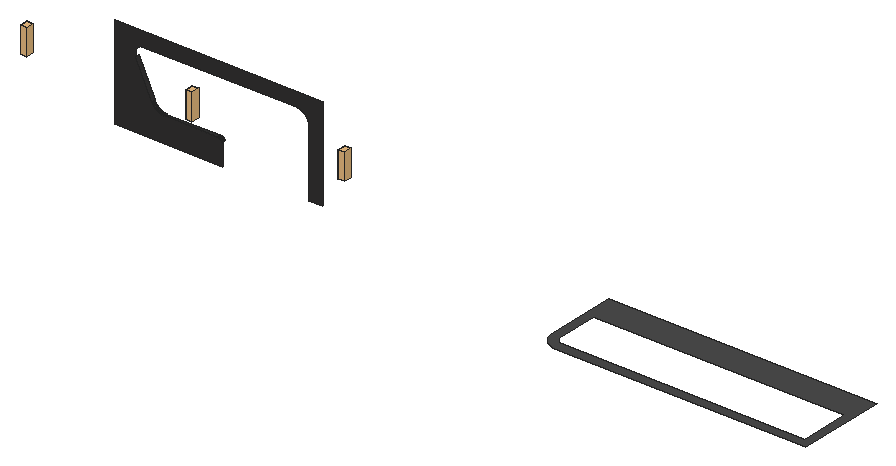
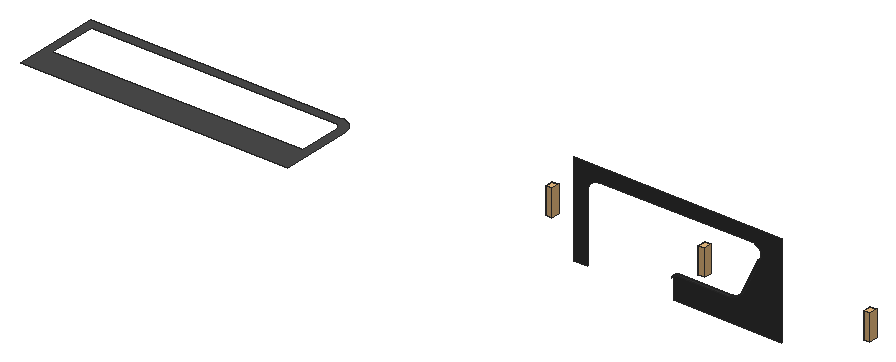
# SketchUp Ruby script. Lengths in inches.
U = 1.inch
M = Sketchup.active_model
def pt(a) = Geom::Point3d.new(a.map { |v| v * U })
def face(e, loops, mat)
  f = e.add_face(loops[0].map { |a| pt(a) })
  loops[1..].each { |l| e.add_face(l.map { |a| pt(a) }).erase! }
  f.material = f.back_material = mat if mat
  f
end
# faces: each face lists its corners as indices into pts; further lists are holes
def faces(e, pts, list, mat = nil) = list.each { |f| face(e, (f[0].is_a?(Array) ? f : [f]).map { |l| l.map { |i| pts[i] } }, mat) }
# xy, xz, yz: faces in a plane at the given z, y or x. An outline is a flat list of corners, or four numbers for a rectangle; further outlines are holes
def ring(l) = l.size == 4 ? [[l[0], l[1]], [l[2], l[1]], [l[2], l[3]], [l[0], l[3]]] : l.each_slice(2).to_a
def flat(e, list, mat, &to3) = list.each { |f| face(e, (f[0].is_a?(Array) ? f : [f]).map { |l| ring(l).map { |u, v| to3.(u, v) } }, mat) }
def xy(e, z, list, mat = nil) = flat(e, list, mat) { |x, y| [x, y, z] }
def xz(e, y, list, mat = nil) = flat(e, list, mat) { |x, z| [x, y, z] }
def yz(e, x, list, mat = nil) = flat(e, list, mat) { |y, z| [x, y, z] }
def lines(e, pts, list) = list.each { |a, b| e.add_line(pt(pts[a]), pt(pts[b])) }
# prism: a flat outline (further loops are holes) pulled along v
def prism(e, loops, v, mat = nil)
  f = face(e, loops, mat); d = Geom::Vector3d.new(v.map { |x| x * U })
  f.pushpull(f.normal.samedirection?(d) ? d.length : -d.length)
end
def box(e, o, s, mat = nil) = prism(e, [[o, [o[0] + s[0], o[1], o[2]], [o[0] + s[0], o[1] + s[1], o[2]], [o[0], o[1] + s[1], o[2]]]], [0, 0, s[2]], mat)
def at(x, y, z, deg = 0) = Geom::Transformation.translation(pt([x, y, z])) * Geom::Transformation.rotation(ORIGIN, Z_AXIS, deg.degrees)
def axes(o, x, y, z) = Geom::Transformation.new([*x, 0, *y, 0, *z, 0, *pt(o).to_a, 1])
def part(name) = M.definitions.add(name)
# library, detail: a bought-in or finely detailed component or shape, given as its bounding box
def library(name, o, s) = part(name).tap { |d| box(d.entities, o, s) }
def detail(e, o, s) = box(e.add_group.entities, o, s)
def put(e, d, t, mat = nil) = e.add_instance(d, t).tap { |i| i.material = mat if mat }
def group(e, t, mat = nil) = e.add_group.tap { |g| g.transformation = t; g.material = mat if mat }.entities
root = M.entities
M.materials.add("[Granite Dark Gray]").color = [51, 50, 50]
M.materials.add("[Stone Coursed Rough]").color = [76, 76, 76]
c1 = library("WALL LIGHT 69",[4.19,4.05,-9.63],[4.61,5.7,18.83])
xy(root,6,[[[479.6875,0,660,0,660,63,468,63,468,11.6875,468.01,11.53,468.02,11.37,468.03,11.22,468.05,10.9,468.07,10.75,468.08,10.59,468.1,10.43,468.125,10.28,468.15,10.12,468.17,9.97,468.2,9.8125,468.23,9.66,468.26,9.51,468.3,9.35,468.33,9.2,468.37,9.05,468.41,8.89,468.49,8.59,468.64,8.14,468.6875,7.99,468.74,7.85,468.8,7.7,468.85,7.55,468.91,7.41,468.97,7.26,469.04,7.12,469.1,6.98,469.17,6.83,469.45,6.27,469.53,6.14,469.61,6,469.6875,5.86,469.77,5.73,469.85,5.6,469.9375,5.46,470.02,5.33,470.2,5.07,470.29,4.95,470.38,4.82,470.48,4.69,470.58,4.57,470.67,4.45,470.77,4.33,470.98,4.09,471.08,3.97,471.1875,3.85,471.3,3.74,471.4,3.625,471.51,3.51,471.625,3.4,471.74,3.3,471.85,3.1875,471.97,3.08,472.09,2.98,472.33,2.77,472.45,2.67,472.57,2.58,472.69,2.48,472.82,2.38,472.95,2.29,473.07,2.2,473.33,2.02,473.46,1.9375,473.6,1.85,473.73,1.77,473.86,1.6875,474,1.61,474.14,1.53,474.27,1.45,474.83,1.17,474.98,1.1,475.12,1.04,475.26,0.97,475.41,0.91,475.55,0.85,475.7,0.8,475.85,0.74,475.99,0.6875,476.14,0.64,476.59,0.49,476.89,0.41,477.05,0.37,477.2,0.33,477.35,0.3,477.51,0.26,477.66,0.23,477.8125,0.2,477.97,0.17,478.12,0.15,478.28,0.125,478.43,0.1,478.59,0.08,478.75,0.07,478.9,0.05,479.22,0.03,479.37,0.02,479.53,0.01],[479.76,6,479.6875,6.01,479.61,6.01,479.45,6.03,479.37,6.03,479.29,6.04,479.22,6.05,479.14,6.0625,479.0625,6.07,478.98,6.09,478.91,6.1,478.83,6.12,478.75,6.13,478.68,6.15,478.6,6.17,478.52,6.18,478.45,6.2,478.37,6.23,478.3,6.25,478.22,6.27,478.15,6.29,478.07,6.32,478,6.34,477.92,6.37,477.78,6.43,477.7,6.46,477.42,6.58,477.35,6.62,477.28,6.65,477.07,6.77,477,6.8,476.93,6.84,476.87,6.88,476.8,6.93,476.73,6.97,476.67,7.01,476.6,7.06,476.54,7.1,476.47,7.15,476.41,7.19,476.29,7.29,476.22,7.34,476.16,7.39,476.1,7.4375,476.04,7.49,475.99,7.54,475.93,7.59,475.87,7.65,475.8125,7.7,475.76,7.76,475.7,7.8125,475.65,7.87,475.59,7.93,475.54,7.99,475.49,8.04,475.4375,8.1,475.39,8.16,475.34,8.22,475.29,8.29,475.19,8.41,475.15,8.47,475.1,8.54,475.06,8.6,475.01,8.67,474.97,8.73,474.93,8.8,474.88,8.87,474.84,8.93,474.8,9,474.77,9.07,474.65,9.28,474.62,9.35,474.58,9.42,474.46,9.7,474.43,9.78,474.37,9.92,474.34,10,474.32,10.07,474.29,10.15,474.27,10.22,474.25,10.3,474.23,10.37,474.2,10.45,474.18,10.52,474.17,10.6,474.15,10.68,474.13,10.75,474.12,10.83,474.1,10.91,474.09,10.98,474.07,11.0625,474.0625,11.14,474.05,11.22,474.04,11.29,474.03,11.37,474.03,11.45,474.01,11.61,474.01,11.6875,474,11.76,474,42,654,42,654,6]]],"[Stone Coursed Rough]")
xy(root,23.99,[[200.21,46,200.3125,48]],"[Granite Dark Gray]")
xy(root,24,[[162,46,200,48],[200,46,200.1,48]],"[Granite Dark Gray]")
xz(root,46,[[126,6,204,6,204,20.1,203.99,20.21,203.99,20.3125,203.98,20.42,203.97,20.52,203.93,20.73,203.89,20.93,203.86,21.04,203.84,21.14,203.8,21.24,203.77,21.34,203.73,21.43,203.7,21.53,203.65,21.625,203.61,21.72,203.5625,21.82,203.52,21.91,203.46,22,203.41,22.09,203.35,22.18,203.3,22.27,203.24,22.35,203.17,22.44,203.11,22.52,202.97,22.68,202.9,22.75,202.83,22.83,202.75,22.9,202.68,22.97,202.52,23.11,202.44,23.17,202.35,23.24,202.27,23.3,202.18,23.35,202.09,23.41,202,23.46,201.91,23.52,201.82,23.5625,201.72,23.61,201.625,23.65,201.53,23.7,201.43,23.73,201.34,23.77,201.24,23.8,201.14,23.84,201.04,23.86,200.93,23.89,200.73,23.93,200.52,23.97,200.42,23.98,200.3125,23.99,200.21,23.99,200.1,24,162,24,161.81,24.01,161.63,24.03,161.44,24.05,161.26,24.07,161.08,24.1,160.89,24.13,160.71,24.16,160.35,24.24,160.16,24.28,159.98,24.33,159.8,24.375,159.625,24.43,159.45,24.48,159.27,24.54,159.1,24.6,158.92,24.67,158.41,24.88,158.07,25.04,157.91,25.125,157.74,25.21,157.42,25.39,157.1,25.59,156.94,25.6875,156.79,25.79,156.64,25.9,156.48,26.01,156.34,26.12,156.19,26.23,156.05,26.35,155.9,26.47,155.76,26.59,155.625,26.72,155.49,26.84,155.36,26.97,155.22,27.1,155.1,27.24,154.97,27.375,154.85,27.51,154.72,27.65,154.61,27.8,154.49,27.94,154.375,28.09,154.27,28.24,154.05,28.54,153.85,28.86,153.75,29.01,153.66,29.17,153.57,29.34,153.48,29.5,153.39,29.67,153.31,29.83,153.23,30,141.69,55,141.54,55.36,141.49,55.49,141.45,55.61,141.41,55.74,141.375,55.86,141.34,55.99,141.3125,56.12,141.28,56.25,141.2,56.77,141.17,57.16,141.17,57.56,141.18,57.6875,141.1875,57.82,141.2,57.95,141.21,58.08,141.27,58.47,141.36,58.86,141.4,58.98,141.4375,59.11,141.48,59.23,141.52,59.36,141.67,59.72,141.85,60.08,141.91,60.19,141.98,60.3,142.05,60.42,142.19,60.64,142.27,60.74,142.35,60.85,142.51,61.05,142.6,61.15,142.6875,61.25,142.78,61.34,142.87,61.4375,142.97,61.53,143.06,61.62,143.16,61.7,143.26,61.79,143.37,61.87,143.47,61.95,143.58,62.03,143.6875,62.1,143.8,62.17,144.02,62.31,144.14,62.375,144.25,62.4375,144.37,62.49,144.49,62.55,144.73,62.65,144.86,62.7,144.98,62.75,145.1,62.79,145.23,62.83,145.36,62.86,145.48,62.9,145.61,62.93,145.74,62.95,145.87,62.98,146,63,257.16,63,257.3125,62.99,257.47,62.99,257.63,62.98,257.78,62.97,258.1,62.93,258.25,62.91,258.41,62.89,258.5625,62.86,258.72,62.83,259.02,62.77,259.18,62.73,259.63,62.61,260.08,62.46,260.23,62.4,260.37,62.34,260.52,62.28,260.8,62.16,260.95,62.09,261.23,61.95,261.36,61.87,261.64,61.71,261.9,61.55,262.29,61.28,262.42,61.1875,262.54,61.09,262.66,60.99,262.79,60.89,262.9,60.79,263.02,60.6875,263.14,60.58,263.58,60.14,263.6875,60.02,263.79,59.9,263.89,59.79,263.99,59.66,264.09,59.54,264.1875,59.42,264.28,59.29,264.55,58.9,264.71,58.64,264.87,58.36,264.95,58.23,265.09,57.95,265.16,57.8,265.28,57.52,265.34,57.37,265.4,57.23,265.46,57.08,265.61,56.63,265.73,56.18,265.77,56.02,265.83,55.72,265.86,55.5625,265.89,55.41,265.91,55.25,265.93,55.1,265.97,54.78,265.98,54.63,265.99,54.47,265.99,54.3125,266,54.16,266,6,276,6,276,73,126,73]],"[Granite Dark Gray]")
p = [[203.7,46,21.53],[203.73,46,21.43],[203.73,48,21.43],[203.7,48,21.53],[203.65,46,21.625],[203.65,48,21.625],
  [203.61,46,21.72],[203.61,48,21.72],[203.5625,46,21.82],[203.5625,48,21.82],[203.52,46,21.91],[203.52,48,21.91],
  [203.46,46,22],[203.46,48,22],[203.41,46,22.09],[203.41,48,22.09],[203.35,46,22.18],[203.35,48,22.18],
  [203.3,46,22.27],[203.3,48,22.27],[203.24,46,22.35],[203.24,48,22.35],[203.11,46,22.52],[203.17,46,22.44],
  [203.17,48,22.44],[203.11,48,22.52],[203.04,46,22.6],[203.04,48,22.6],[202.97,46,22.68],[202.97,48,22.68],
  [202.9,46,22.75],[202.9,48,22.75],[202.75,46,22.9],[202.83,46,22.83],[202.83,48,22.83],[202.75,48,22.9],
  [202.68,46,22.97],[202.68,48,22.97],[202.52,46,23.11],[202.6,46,23.04],[202.6,48,23.04],[202.52,48,23.11],
  [202.44,46,23.17],[202.44,48,23.17],[202.27,46,23.3],[202.35,46,23.24],[202.35,48,23.24],[202.27,48,23.3],
  [202.18,46,23.35],[202.18,48,23.35],[202,46,23.46],[202.09,46,23.41],[202.09,48,23.41],[202,48,23.46],
  [201.82,46,23.5625],[201.91,46,23.52],[201.91,48,23.52],[201.82,48,23.5625],[201.625,46,23.65],[201.72,46,23.61],
  [201.72,48,23.61],[201.625,48,23.65],[201.34,46,23.77],[201.43,46,23.73],[201.43,48,23.73],[201.34,48,23.77],
  [201.53,46,23.7],[201.53,48,23.7],[201.04,46,23.86],[201.14,46,23.84],[201.14,48,23.84],[201.04,48,23.86],
  [201.24,46,23.8],[201.24,48,23.8],[200.625,46,23.95],[200.73,46,23.93],[200.73,48,23.93],[200.625,48,23.95],
  [200.83,46,23.91],[200.83,48,23.91],[200.93,46,23.89],[200.93,48,23.89],[161.44,46,24.05],[161.26,46,24.07],
  [161.26,48,24.07],[161.44,48,24.05],[161.63,46,24.03],[161.63,48,24.03],[161.81,46,24.01],[161.81,48,24.01],
  [162,46,24],[162,48,24],[200.1,46,24],[200.21,46,23.99],[200.21,48,23.99],[200.1,48,24],
  [200.3125,46,23.99],[200.42,46,23.98],[200.42,48,23.98],[200.3125,48,23.99],[200.52,46,23.97],[200.52,48,23.97],
  [160.89,46,24.13],[160.71,46,24.16],[160.71,48,24.16],[160.89,48,24.13],[161.08,46,24.1],[161.08,48,24.1],
  [160.35,46,24.24],[160.16,46,24.28],[160.16,48,24.28],[160.35,48,24.24],[160.53,46,24.2],[160.53,48,24.2],
  [159.98,46,24.33],[159.8,46,24.375],[159.8,48,24.375],[159.98,48,24.33],[159.625,46,24.43],[159.45,46,24.48],
  [159.45,48,24.48],[159.625,48,24.43],[159.27,46,24.54],[159.1,46,24.6],[159.1,48,24.6],[159.27,48,24.54],
  [158.92,46,24.67],[158.92,48,24.67],[158.75,46,24.74],[158.58,46,24.81],[158.58,48,24.81],[158.75,48,24.74],
  [158.41,46,24.88],[158.41,48,24.88],[158.24,46,24.96],[158.24,48,24.96],[158.07,46,25.04],[157.91,46,25.125],
  [157.91,48,25.125],[158.07,48,25.04],[157.74,46,25.21],[157.74,48,25.21],[157.58,46,25.3],[157.58,48,25.3],
  [157.42,46,25.39],[157.42,48,25.39],[157.26,46,25.49],[157.26,48,25.49],[157.1,46,25.59],[157.1,48,25.59],
  [156.94,46,25.6875],[156.94,48,25.6875],[156.79,46,25.79],[156.79,48,25.79],[156.64,46,25.9],[156.64,48,25.9],
  [156.48,46,26.01],[156.48,48,26.01],[156.34,46,26.12],[156.34,48,26.12],[156.19,46,26.23],[156.19,48,26.23],
  [156.05,46,26.35],[156.05,48,26.35],[155.9,46,26.47],[155.9,48,26.47],[155.76,46,26.59],[155.76,48,26.59],
  [155.625,46,26.72],[155.625,48,26.72],[155.49,46,26.84],[155.49,48,26.84],[155.36,46,26.97],[155.36,48,26.97],
  [155.22,46,27.1],[155.22,48,27.1],[155.1,46,27.24],[155.1,48,27.24],[154.97,46,27.375],[154.97,48,27.375],
  [154.85,46,27.51],[154.85,48,27.51],[154.72,46,27.65],[154.72,48,27.65],[154.61,46,27.8],[154.61,48,27.8],
  [154.49,46,27.94],[154.49,48,27.94],[154.375,46,28.09],[154.375,48,28.09],[154.27,46,28.24],[154.27,48,28.24],
  [154.16,46,28.39],[154.16,48,28.39],[154.05,46,28.54],[154.05,48,28.54],[153.95,46,28.7],[153.95,48,28.7],
  [153.85,46,28.86],[153.85,48,28.86],[153.75,46,29.01],[153.75,48,29.01],[153.66,46,29.17],[153.66,48,29.17],
  [153.57,46,29.34],[153.57,48,29.34],[153.48,46,29.5],[153.48,48,29.5],[153.39,46,29.67],[153.39,48,29.67],
  [153.31,46,29.83],[153.31,48,29.83],[153.23,46,30],[153.23,48,30],[141.69,48,55],[141.69,46,55],
  [156,46,24],[156,48,24]]
faces(root,p,[[0,1,2,3],[4,0,3,5],[6,4,5,7],[8,6,7,9],[10,8,9,11],[12,10,11,13],[14,12,13,15],[16,14,15,17],
  [18,16,17,19],[20,18,19,21],[22,23,24,25],[23,20,21,24],[26,22,25,27],[28,26,27,29],[30,28,29,31],[32,33,34,35],
  [33,30,31,34],[36,32,35,37],[38,39,40,41],[39,36,37,40],[42,38,41,43],[44,45,46,47],[45,42,43,46],[48,44,47,49],
  [50,51,52,53],[51,48,49,52],[54,55,56,57],[55,50,53,56],[58,59,60,61],[59,54,57,60],[62,63,64,65],[63,66,67,64],
  [66,58,61,67],[68,69,70,71],[69,72,73,70],[72,62,65,73],[74,75,76,77],[75,78,79,76],[78,80,81,79],[80,68,71,81],
  [82,83,84,85],[86,82,85,87],[88,86,87,89],[90,88,89,91],[92,93,94,95],[96,97,98,99],[97,100,101,98],[100,74,77,101],
  [102,103,104,105],[106,102,105,107],[83,106,107,84],[108,109,110,111],[112,108,111,113],[103,112,113,104],[114,115,116,117],[109,114,117,110],
  [118,119,120,121],[115,118,121,116],[122,123,124,125],[119,122,125,120],[123,126,127,124],[128,129,130,131],[126,128,131,127],[129,132,133,130],
  [132,134,135,133],[136,137,138,139],[134,136,139,135],[137,140,141,138],[140,142,143,141],[142,144,145,143],[144,146,147,145],[146,148,149,147],
  [148,150,151,149],[150,152,153,151],[152,154,155,153],[154,156,157,155],[156,158,159,157],[158,160,161,159],[160,162,163,161],[162,164,165,163],
  [164,166,167,165],[166,168,169,167],[168,170,171,169],[170,172,173,171],[172,174,175,173],[174,176,177,175],[176,178,179,177],[178,180,181,179],
  [180,182,183,181],[182,184,185,183],[184,186,187,185],[186,188,189,187],[188,190,191,189],[190,192,193,191],[192,194,195,193],[194,196,197,195],
  [196,198,199,197],[198,200,201,199],[200,202,203,201],[202,204,205,203],[204,206,207,205],[206,208,209,207],[208,210,211,209],[210,212,213,211],
  [213,214,215,212]],"[Granite Dark Gray]")
lines(root,p,[[216,217]])
put(root,c1,at(57.2,38.25,39.5625))
put(root,c1,at(176.03,38.25,39.5625))
put(root,c1,at(285.72,38.25,39.5625))
